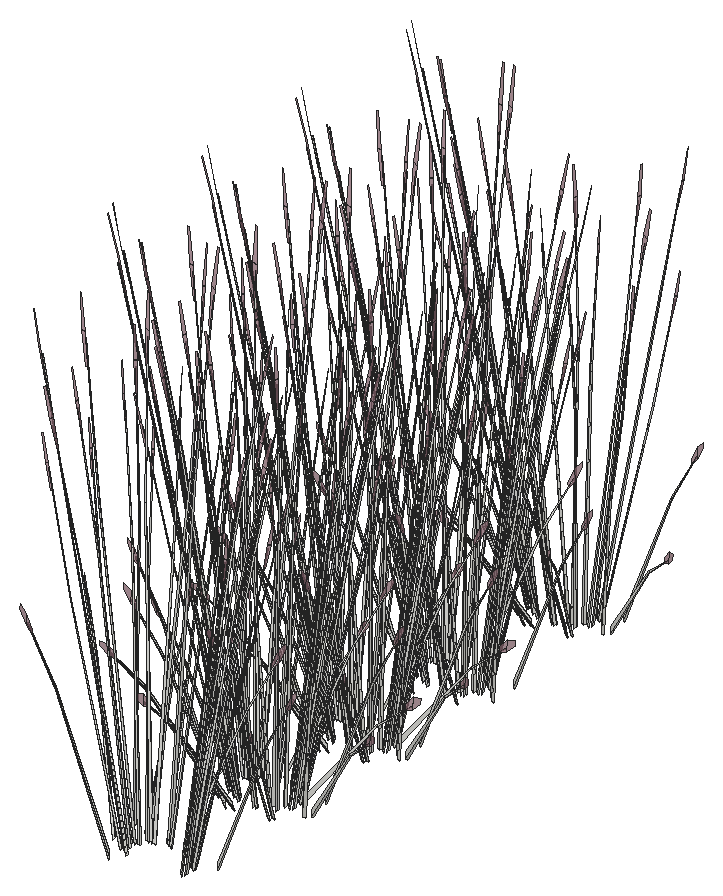
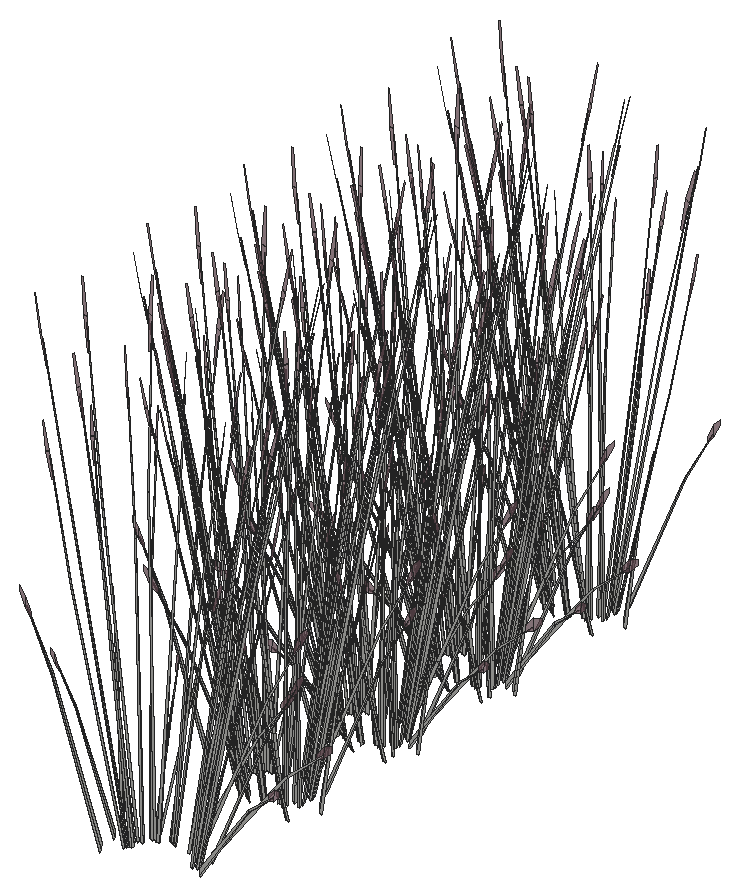
# SketchUp Ruby script. Lengths in inches.
U = 1.inch
M = Sketchup.active_model
def pt(a) = Geom::Point3d.new(a.map { |v| v * U })
def face(e, loops, mat)
  f = e.add_face(loops[0].map { |a| pt(a) })
  loops[1..].each { |l| e.add_face(l.map { |a| pt(a) }).erase! }
  f.material = f.back_material = mat if mat
  f
end
# faces: each face lists its corners as indices into pts; further lists are holes
def faces(e, pts, list, mat = nil) = list.each { |f| face(e, (f[0].is_a?(Array) ? f : [f]).map { |l| l.map { |i| pts[i] } }, mat) }
# xy, xz, yz: faces in a plane at the given z, y or x. An outline is a flat list of corners, or four numbers for a rectangle; further outlines are holes
def ring(l) = l.size == 4 ? [[l[0], l[1]], [l[2], l[1]], [l[2], l[3]], [l[0], l[3]]] : l.each_slice(2).to_a
def flat(e, list, mat, &to3) = list.each { |f| face(e, (f[0].is_a?(Array) ? f : [f]).map { |l| ring(l).map { |u, v| to3.(u, v) } }, mat) }
def xy(e, z, list, mat = nil) = flat(e, list, mat) { |x, y| [x, y, z] }
def xz(e, y, list, mat = nil) = flat(e, list, mat) { |x, z| [x, y, z] }
def yz(e, x, list, mat = nil) = flat(e, list, mat) { |y, z| [x, y, z] }
def lines(e, pts, list) = list.each { |a, b| e.add_line(pt(pts[a]), pt(pts[b])) }
# prism: a flat outline (further loops are holes) pulled along v
def prism(e, loops, v, mat = nil)
  f = face(e, loops, mat); d = Geom::Vector3d.new(v.map { |x| x * U })
  f.pushpull(f.normal.samedirection?(d) ? d.length : -d.length)
end
def box(e, o, s, mat = nil) = prism(e, [[o, [o[0] + s[0], o[1], o[2]], [o[0] + s[0], o[1] + s[1], o[2]], [o[0], o[1] + s[1], o[2]]]], [0, 0, s[2]], mat)
def at(x, y, z, deg = 0) = Geom::Transformation.translation(pt([x, y, z])) * Geom::Transformation.rotation(ORIGIN, Z_AXIS, deg.degrees)
def axes(o, x, y, z) = Geom::Transformation.new([*x, 0, *y, 0, *z, 0, *pt(o).to_a, 1])
def part(name) = M.definitions.add(name)
# library, detail: a bought-in or finely detailed component or shape, given as its bounding box
def library(name, o, s) = part(name).tap { |d| box(d.entities, o, s) }
def detail(e, o, s) = box(e.add_group.entities, o, s)
def put(e, d, t, mat = nil) = e.add_instance(d, t).tap { |i| i.material = mat if mat }
def group(e, t, mat = nil) = e.add_group.tap { |g| g.transformation = t; g.material = mat if mat }.entities
root = M.entities
M.materials.add("LightPink_Translucent").color = [144, 107, 117]
M.materials["LightPink_Translucent"].alpha = 0.75
c1 = part("blade")
p = [[2.15,0.21,22],[0,0.17,0],[0.09,0.45,0],[2.18,0.31,22],[2.29,0.31,22],[0.38,0.45,0],
  [2.48,0.24,33],[2.49,0.24,33],[2.48,0.22,33]]
faces(c1.entities,p,[[0,1,2,3],[4,5,2,3],[6,3,4,7],[8,0,3,6]])
c2 = part("seeds")
p = [[0.3,-0.1,1.38],[-0.01,-0.03,1.59],[-0.01,-0.03,0.03],[0.14,-0.07,-0.07],[0.29,-0.03,3],[0.15,0.01,3.11]]
faces(c2.entities,p,[[0,1,2,3],[1,0,4,5]],"LightPink_Translucent")
c3 = part("blade with seeds")
put(c3.entities,c1,at(0,0,0))
put(c3.entities,c2,axes([2.4,0.25,30.99],[1.5799,-0.05474,1.17369],[-0.12525,1.92788,0.29478],[-0.07173,-0.02425,1.56792]))
put(root,c3,axes([336.16,386.52,52.18],[0.34663,0.16434,0.05682],[-0.20181,0.23402,0.44729],[0.11113,-0.07566,0.68204]))
put(root,c3,axes([336.0625,386.45,52.18],[0.12522,0.35963,0.42415],[-0.49122,0.06241,0.34973],[0.14477,-0.08458,0.87768]))
put(root,c3,axes([331.47,385.46,52.16],[0.03743,0.039,1.56736],[-0.18045,0.35054,-0.1481],[-0.18276,0.00254,0.27737]))
put(root,c3,axes([332.25,386.07,52.46],[0.28729,0.24465,0.31292],[-0.32804,0.23159,-0.40398],[-0.16667,-0.03524,0.77298]))
put(root,c3,axes([335.83,387.33,52.46],[-0.41962,-0.10901,0.31292],[0.12239,-0.31802,-0.40398],[0.16894,-0.02916,0.77298]))
put(root,c3,axes([331.4375,386.75,52.18],[0.14265,-0.35629,0.42415],[0.46898,0.12183,0.34973],[-0.18443,0.02141,0.87768]))
put(root,c3,axes([331.4,386.66,52.18],[-0.18545,-0.26643,0.05682],[0.33817,-0.13041,0.44729],[-0.14907,0.02573,0.68204]))
put(root,c3,axes([336.21,387.43,52.18],[0.18545,0.26643,0.05682],[-0.33817,0.13041,0.44729],[0.14907,-0.02573,0.68204]))
put(root,c3,axes([336.18,387.34,52.18],[-0.14265,0.35629,0.42415],[-0.46898,-0.12183,0.34973],[0.18443,-0.02141,0.87768]))
put(root,c3,axes([331.78,386.76,52.46],[0.41962,0.10901,0.31292],[-0.12239,0.31802,-0.40398],[-0.16894,0.02916,0.77298]))
put(root,c3,axes([337.02,388.49,52.16],[-0.04566,-0.03421,1.56736],[0.09987,-0.36669,-0.1481],[0.17984,-0.02343,0.27737]))
put(root,c3,axes([335.36,388.02,52.46],[-0.28729,-0.24465,0.31292],[0.32804,-0.23159,-0.40398],[0.16667,0.03524,0.77298]))
put(root,c3,axes([331.55,387.64,52.18],[-0.12522,-0.35963,0.42415],[0.49122,-0.06241,0.34973],[-0.14477,0.08458,0.87768]))
put(root,c3,axes([331.45,387.57,52.18],[-0.34663,-0.16434,0.05682],[0.20181,-0.23402,0.44729],[-0.11113,0.07566,0.68204]))
put(root,c3,axes([331.85,387.52,52.46],[0.43951,-0.05584,0.31292],[0.11606,0.31924,-0.40398],[-0.12595,0.08575,0.77298]))
put(root,c3,axes([330.16,387.38,52.16],[0.06444,0.01048,1.56736],[0.19934,0.34525,-0.1481],[-0.13191,0.09062,0.27737]))
put(root,c3,axes([335.62,388.24,52.18],[-0.02542,0.29714,0.05682],[-0.38391,-0.00815,0.44729],[0.14706,0.03109,0.68204]))
put(root,c3,axes([335.65,388.15,52.18],[-0.3723,0.25748,0.42415],[-0.32109,-0.27343,0.34973],[0.17467,0.04749,0.87768]))
put(root,c3,axes([330.85,388.43,52.99],[0.44556,0.1043,-0.05733],[-0.13706,0.32103,-0.25992],[-0.07288,0.04874,0.85731]))
put(root,c3,axes([334.47,388.45,52.46],[-0.07798,-0.31474,0.31292],[0.44579,-0.08311,-0.40398],[0.11974,0.09019,0.77298]))
put(root,c3,axes([332.45,388.16,52.46],[0.34164,-0.20573,0.31292],[0.3234,0.23491,-0.40398],[-0.04921,0.11936,0.77298]))
put(root,c3,axes([334.04,388.89,52.16],[0.00149,-0.04731,1.56736],[0.4327,-0.20872,-0.1481],[0.1503,0.0745,0.27737]))
put(root,c3,axes([332.14,388.34,52.18],[-0.41493,-0.01821,0.05682],[0.01138,-0.27493,0.44729],[-0.04342,0.10531,0.68204]))
put(root,c3,axes([332.27,388.37,52.18],[-0.35954,-0.26661,0.42415],[0.38183,-0.22994,0.34973],[-0.06632,0.12508,0.87768]))
put(root,c3,axes([333.4,388.5,52.46],[0.15222,-0.30049,0.31292],[0.44409,0.08764,-0.40398],[0.04072,0.12098,0.77298]))
put(root,c3,axes([334.54,388.73,52.18],[-0.22948,0.24822,0.05682],[-0.32679,-0.14452,0.44729],[0.10565,0.07958,0.68204]))
put(root,c3,axes([334,389.57,52.99],[0.34892,-0.22417,-0.05733],[0.3197,0.24551,-0.25992],[0.02251,0.06957,0.85731]))
put(root,c3,axes([334.64,388.66,52.18],[-0.5022,0.08967,0.42415],[-0.08716,-0.35177,0.34973],[0.11811,0.10367,0.87768]))
put(root,c3,axes([333.27,388.77,52.18],[-0.37205,0.1328,0.05682],[-0.18211,-0.24217,0.44729],[0.03593,0.10675,0.68204]))
put(root,c3,axes([332.23,388.21,52.77],[0.55492,0.01936,-0.11927],[-0.01517,0.36657,-0.66198],[-0.03855,0.14118,1.00587]))
put(root,c3,axes([333.4,388.74,52.47],[-0.49753,-0.10215,0.47081],[0.17013,-0.33585,0.3882],[0.0299,0.13207,0.97422]))
put(root,c3,axes([331.05,389.18,52.16],[0.05728,-0.02359,1.56736],[0.47345,0.15692,-0.1481],[-0.01113,0.13066,0.27737]))
put(root,c3,axes([333.57,394.3,52.17],[-0.07723,-0.05479,1.54581],[-0.51538,0.03473,-0.24447],[-0.08225,-0.13104,0.12397]))
put(root,c3,axes([335.89,394.98,52.17],[-0.00487,-0.07777,1.54581],[-0.41166,-0.22476,-0.24447],[0.06364,-0.13625,0.12397]))
put(root,c3,axes([335.78,394.7,52.16],[-0.05128,0.02985,1.56736],[-0.5024,-0.1007,-0.1481],[-0.01819,-0.13025,0.27737]))
put(root,c3,axes([333.05,394.125,52.16],[-0.00942,0.04684,1.56736],[-0.46458,0.16998,-0.1481],[-0.13671,-0.08689,0.27737]))
put(root,c3,axes([332.94,394.96,52.5],[0.56246,-0.10044,0.47505],[0.09762,0.39398,0.3917],[-0.13228,-0.11611,0.983]))
put(root,c3,axes([334.22,395.03,52.18],[0.49753,0.10215,0.42415],[-0.17013,0.33585,0.34973],[-0.0299,-0.13207,0.87768]))
put(root,c3,axes([334.35,395,52.18],[0.37205,-0.1328,0.05682],[0.18211,0.24217,0.44729],[-0.03593,-0.10675,0.68204]))
put(root,c3,axes([333.07,395.04,52.18],[0.22948,-0.24822,0.05682],[0.32679,0.14452,0.44729],[-0.10565,-0.07958,0.68204]))
put(root,c3,axes([334.21,395.28,52.46],[-0.15222,0.30049,0.31292],[-0.44409,-0.08764,-0.40398],[-0.04072,-0.12098,0.77298]))
put(root,c3,axes([335.34,395.4,52.18],[0.35954,0.26661,0.42415],[-0.38183,0.22994,0.34973],[0.06632,-0.12508,0.87768]))
put(root,c3,axes([333.18,395.02,52.8],[-0.33698,0.3746,-0.12034],[-0.48801,-0.21581,-0.66795],[-0.16964,-0.10584,1.01494]))
put(root,c3,axes([335.48,395.43,52.18],[0.41493,0.01821,0.05682],[-0.01138,0.27493,0.44729],[0.04342,-0.10531,0.68204]))
put(root,c3,axes([335.17,395.62,52.46],[-0.34164,0.20573,0.31292],[-0.3234,-0.23491,-0.40398],[0.04921,-0.11936,0.77298]))
put(root,c3,axes([331.88,394.91,52.17],[-0.10864,-0.00276,1.54581],[-0.34587,0.27582,-0.24447],[-0.18454,-0.05636,0.12397]))
put(root,c3,axes([333.14,395.33,52.46],[0.07798,0.31474,0.31292],[-0.44579,0.08311,-0.40398],[-0.11974,-0.09019,0.77298]))
put(root,c3,axes([331.8,395.53,52.5],[0.41698,-0.28837,0.47505],[0.35962,0.30624,0.3917],[-0.19563,-0.05319,0.983]))
put(root,c3,axes([337.14,396.1875,52.16],[-0.06595,-0.00297,1.56736],[-0.27386,-0.31799,-0.1481],[0.10998,-0.10455,0.27737]))
put(root,c3,axes([331.99,395.53,52.18],[0.02542,-0.29714,0.05682],[0.38391,0.00815,0.44729],[-0.14706,-0.03109,0.68204]))
put(root,c3,axes([335.76,396.25,52.46],[-0.43951,0.05584,0.31292],[-0.11606,-0.31924,-0.40398],[0.12595,-0.08575,0.77298]))
put(root,c3,axes([336.16,396.2,52.18],[0.34663,0.16434,0.05682],[-0.20181,0.23402,0.44729],[0.11113,-0.07566,0.68204]))
put(root,c3,axes([336.0625,396.13,52.18],[0.12522,0.35963,0.42415],[-0.49122,0.06241,0.34973],[0.14477,-0.08458,0.87768]))
put(root,c3,axes([337.39,396.57,52.17],[0.07006,-0.05952,1.54581],[-0.08968,-0.3651,-0.24447],[0.1758,-0.06922,0.12397]))
put(root,c3,axes([331.47,395.14,52.16],[0.03743,0.039,1.56736],[-0.18045,0.35054,-0.1481],[-0.18276,0.00254,0.27737]))
put(root,c3,axes([332.25,395.75,52.46],[0.28729,0.24465,0.31292],[-0.32804,0.23159,-0.40398],[-0.16667,-0.03524,0.77298]))
put(root,c3,axes([335.83,397.01,52.46],[-0.41962,-0.10901,0.31292],[0.12239,-0.31802,-0.40398],[0.16894,-0.02916,0.77298]))
put(root,c3,axes([331.4375,396.43,52.18],[0.14265,-0.35629,0.42415],[0.46898,0.12183,0.34973],[-0.18443,0.02141,0.87768]))
put(root,c3,axes([331.4,396.34,52.18],[-0.18545,-0.26643,0.05682],[0.33817,-0.13041,0.44729],[-0.14907,0.02573,0.68204]))
put(root,c3,axes([336.21,397.11,52.18],[0.18545,0.26643,0.05682],[-0.33817,0.13041,0.44729],[0.14907,-0.02573,0.68204]))
put(root,c3,axes([336.18,397.02,52.18],[-0.14265,0.35629,0.42415],[-0.46898,-0.12183,0.34973],[0.18443,-0.02141,0.87768]))
put(root,c3,axes([331.78,396.4375,52.46],[0.41962,0.10901,0.31292],[-0.12239,0.31802,-0.40398],[-0.16894,0.02916,0.77298]))
put(root,c3,axes([337.02,398.17,52.16],[-0.04566,-0.03421,1.56736],[0.09987,-0.36669,-0.1481],[0.17984,-0.02343,0.27737]))
put(root,c3,axes([331.08,396.68,52.17],[-0.08245,0.05073,1.54581],[0.00701,0.37067,-0.24447],[-0.18899,0.0482,0.12397]))
put(root,c3,axes([335.36,397.7,52.46],[-0.28729,-0.24465,0.31292],[0.32804,-0.23159,-0.40398],[0.16667,0.03524,0.77298]))
put(root,c3,axes([335.88,397.62,52.17],[0.10831,-0.00661,1.54581],[0.29709,-0.30358,-0.24447],[0.19266,0.04007,0.12397]))
put(root,c3,axes([331.55,397.32,52.18],[-0.12522,-0.35963,0.42415],[0.49122,-0.06241,0.34973],[-0.14477,0.08458,0.87768]))
put(root,c3,axes([331.45,397.25,52.18],[-0.34663,-0.16434,0.05682],[0.20181,-0.23402,0.44729],[-0.11113,0.07566,0.68204]))
put(root,c3,axes([331.85,397.2,52.46],[0.43951,-0.05584,0.31292],[0.11606,0.31924,-0.40398],[-0.12595,0.08575,0.77298]))
put(root,c3,axes([330.16,397.06,52.16],[0.06444,0.01048,1.56736],[0.19934,0.34525,-0.1481],[-0.13191,0.09062,0.27737]))
put(root,c3,axes([335.62,397.92,52.18],[-0.02542,0.29714,0.05682],[-0.38391,-0.00815,0.44729],[0.14706,0.03109,0.68204]))
put(root,c3,axes([335.65,397.83,52.18],[-0.3723,0.25748,0.42415],[-0.32109,-0.27343,0.34973],[0.17467,0.04749,0.87768]))
put(root,c3,axes([330.85,398.11,52.99],[0.44556,0.1043,-0.05733],[-0.13706,0.32103,-0.25992],[-0.07288,0.04874,0.85731]))
put(root,c3,axes([334.47,398.125,52.46],[-0.07798,-0.31474,0.31292],[0.44579,-0.08311,-0.40398],[0.11974,0.09019,0.77298]))
put(root,c3,axes([332.45,397.84,52.46],[0.34164,-0.20573,0.31292],[0.3234,0.23491,-0.40398],[-0.04921,0.11936,0.77298]))
put(root,c3,axes([334.04,398.57,52.16],[0.00149,-0.04731,1.56736],[0.4327,-0.20872,-0.1481],[0.1503,0.0745,0.27737]))
put(root,c3,axes([332.14,398.02,52.18],[-0.41493,-0.01821,0.05682],[0.01138,-0.27493,0.44729],[-0.04342,0.10531,0.68204]))
put(root,c3,axes([332.27,398.05,52.18],[-0.35954,-0.26661,0.42415],[0.38183,-0.22994,0.34973],[-0.06632,0.12508,0.87768]))
put(root,c3,axes([333.4,398.18,52.46],[0.15222,-0.30049,0.31292],[0.44409,0.08764,-0.40398],[0.04072,0.12098,0.77298]))
put(root,c3,axes([334.54,398.41,52.18],[-0.22948,0.24822,0.05682],[-0.32679,-0.14452,0.44729],[0.10565,0.07958,0.68204]))
put(root,c3,axes([334,399.25,52.99],[0.34892,-0.22417,-0.05733],[0.3197,0.24551,-0.25992],[0.02251,0.06957,0.85731]))
put(root,c3,axes([334.64,398.34,52.18],[-0.5022,0.08967,0.42415],[-0.08716,-0.35177,0.34973],[0.11811,0.10367,0.87768]))
put(root,c3,axes([333.57,402.77,52.17],[-0.07723,-0.05479,1.54581],[-0.51538,0.03473,-0.24447],[-0.08225,-0.13104,0.12397]))
put(root,c3,axes([333.27,398.45,52.18],[-0.37205,0.1328,0.05682],[-0.18211,-0.24217,0.44729],[0.03593,0.10675,0.68204]))
put(root,c3,axes([331.09,398.07,52.17],[-0.01255,0.07733,1.54581],[0.35618,0.269,-0.24447],[-0.09325,0.12721,0.12397]))
put(root,c3,axes([332.23,397.89,52.77],[0.55492,0.01936,-0.11927],[-0.01517,0.36657,-0.66198],[-0.03855,0.14118,1.00587]))
put(root,c3,axes([333.4,398.42,52.47],[-0.49753,-0.10215,0.47081],[0.17013,-0.33585,0.3882],[0.0299,0.13207,0.97422]))
put(root,c3,axes([335.89,403.4375,52.17],[-0.00487,-0.07777,1.54581],[-0.41166,-0.22476,-0.24447],[0.06364,-0.13625,0.12397]))
put(root,c3,axes([335.78,403.16,52.16],[-0.05128,0.02985,1.56736],[-0.5024,-0.1007,-0.1481],[-0.01819,-0.13025,0.27737]))
put(root,c3,axes([333.05,402.59,52.16],[-0.00942,0.04684,1.56736],[-0.46458,0.16998,-0.1481],[-0.13671,-0.08689,0.27737]))
put(root,c3,axes([331.05,398.86,52.16],[0.05728,-0.02359,1.56736],[0.47345,0.15692,-0.1481],[-0.01113,0.13066,0.27737]))
put(root,c3,axes([332.94,403.42,52.5],[0.56246,-0.10044,0.47505],[0.09762,0.39398,0.3917],[-0.13228,-0.11611,0.983]))
put(root,c3,axes([334.22,403.49,52.18],[0.49753,0.10215,0.42415],[-0.17013,0.33585,0.34973],[-0.0299,-0.13207,0.87768]))
put(root,c3,axes([334.35,403.47,52.18],[0.37205,-0.1328,0.05682],[0.18211,0.24217,0.44729],[-0.03593,-0.10675,0.68204]))
put(root,c3,axes([333.14,399.03,52.17],[0.064,0.06292,1.54581],[0.51651,0.02472,-0.24447],[0.05194,0.13877,0.12397]))
put(root,c3,axes([333.07,403.5,52.18],[0.22948,-0.24822,0.05682],[0.32679,0.14452,0.44729],[-0.10565,-0.07958,0.68204]))
put(root,c3,axes([334.21,403.74,52.46],[-0.15222,0.30049,0.31292],[-0.44409,-0.08764,-0.40398],[-0.04072,-0.12098,0.77298]))
put(root,c3,axes([335.34,403.87,52.18],[0.35954,0.26661,0.42415],[-0.38183,0.22994,0.34973],[0.06632,-0.12508,0.87768]))
put(root,c3,axes([333.18,403.48,52.8],[-0.33698,0.3746,-0.12034],[-0.48801,-0.21581,-0.66795],[-0.16964,-0.10584,1.01494]))
put(root,c3,axes([335.48,403.89,52.18],[0.41493,0.01821,0.05682],[-0.01138,0.27493,0.44729],[0.04342,-0.10531,0.68204]))
put(root,c3,axes([335.17,404.08,52.46],[-0.34164,0.20573,0.31292],[-0.3234,-0.23491,-0.40398],[0.04921,-0.11936,0.77298]))
put(root,c3,axes([331.88,403.37,52.17],[-0.10864,-0.00276,1.54581],[-0.34587,0.27582,-0.24447],[-0.18454,-0.05636,0.12397]))
put(root,c3,axes([333.14,403.79,52.46],[0.07798,0.31474,0.31292],[-0.44579,0.08311,-0.40398],[-0.11974,-0.09019,0.77298]))
put(root,c3,axes([331.8,403.99,52.5],[0.41698,-0.28837,0.47505],[0.35962,0.30624,0.3917],[-0.19563,-0.05319,0.983]))
put(root,c3,axes([337.14,404.65,52.16],[-0.06595,-0.00297,1.56736],[-0.27386,-0.31799,-0.1481],[0.10998,-0.10455,0.27737]))
put(root,c3,axes([331.99,403.99,52.18],[0.02542,-0.29714,0.05682],[0.38391,0.00815,0.44729],[-0.14706,-0.03109,0.68204]))
put(root,c3,axes([335.76,404.71,52.46],[-0.43951,0.05584,0.31292],[-0.11606,-0.31924,-0.40398],[0.12595,-0.08575,0.77298]))
put(root,c3,axes([336.16,404.66,52.18],[0.34663,0.16434,0.05682],[-0.20181,0.23402,0.44729],[0.11113,-0.07566,0.68204]))
put(root,c3,axes([336.0625,404.59,52.18],[0.12522,0.35963,0.42415],[-0.49122,0.06241,0.34973],[0.14477,-0.08458,0.87768]))
put(root,c3,axes([337.39,405.03,52.17],[0.07006,-0.05952,1.54581],[-0.08968,-0.3651,-0.24447],[0.1758,-0.06922,0.12397]))
put(root,c3,axes([331.47,403.6,52.16],[0.03743,0.039,1.56736],[-0.18045,0.35054,-0.1481],[-0.18276,0.00254,0.27737]))
put(root,c3,axes([332.25,404.21,52.46],[0.28729,0.24465,0.31292],[-0.32804,0.23159,-0.40398],[-0.16667,-0.03524,0.77298]))
put(root,c3,axes([335.83,405.48,52.46],[-0.41962,-0.10901,0.31292],[0.12239,-0.31802,-0.40398],[0.16894,-0.02916,0.77298]))
put(root,c3,axes([331.4375,404.9,52.18],[0.14265,-0.35629,0.42415],[0.46898,0.12183,0.34973],[-0.18443,0.02141,0.87768]))
put(root,c3,axes([331.4,404.8,52.18],[-0.18545,-0.26643,0.05682],[0.33817,-0.13041,0.44729],[-0.14907,0.02573,0.68204]))
put(root,c3,axes([336.21,405.58,52.18],[0.18545,0.26643,0.05682],[-0.33817,0.13041,0.44729],[0.14907,-0.02573,0.68204]))
put(root,c3,axes([336.18,405.48,52.18],[-0.14265,0.35629,0.42415],[-0.46898,-0.12183,0.34973],[0.18443,-0.02141,0.87768]))
put(root,c3,axes([331.78,404.9,52.46],[0.41962,0.10901,0.31292],[-0.12239,0.31802,-0.40398],[-0.16894,0.02916,0.77298]))
put(root,c3,axes([337.02,406.63,52.16],[-0.04566,-0.03421,1.56736],[0.09987,-0.36669,-0.1481],[0.17984,-0.02343,0.27737]))
put(root,c3,axes([331.08,405.15,52.17],[-0.08245,0.05073,1.54581],[0.00701,0.37067,-0.24447],[-0.18899,0.0482,0.12397]))
put(root,c3,axes([335.36,406.16,52.46],[-0.28729,-0.24465,0.31292],[0.32804,-0.23159,-0.40398],[0.16667,0.03524,0.77298]))
put(root,c3,axes([335.88,406.08,52.17],[0.10831,-0.00661,1.54581],[0.29709,-0.30358,-0.24447],[0.19266,0.04007,0.12397]))
put(root,c3,axes([331.55,405.78,52.18],[-0.12522,-0.35963,0.42415],[0.49122,-0.06241,0.34973],[-0.14477,0.08458,0.87768]))
put(root,c3,axes([331.45,405.71,52.18],[-0.34663,-0.16434,0.05682],[0.20181,-0.23402,0.44729],[-0.11113,0.07566,0.68204]))
put(root,c3,axes([331.85,405.66,52.46],[0.43951,-0.05584,0.31292],[0.11606,0.31924,-0.40398],[-0.12595,0.08575,0.77298]))
put(root,c3,axes([330.16,405.52,52.16],[0.06444,0.01048,1.56736],[0.19934,0.34525,-0.1481],[-0.13191,0.09062,0.27737]))
put(root,c3,axes([335.62,406.38,52.18],[-0.02542,0.29714,0.05682],[-0.38391,-0.00815,0.44729],[0.14706,0.03109,0.68204]))
put(root,c3,axes([335.65,406.29,52.18],[-0.3723,0.25748,0.42415],[-0.32109,-0.27343,0.34973],[0.17467,0.04749,0.87768]))
put(root,c3,axes([330.85,406.57,52.99],[0.44556,0.1043,-0.05733],[-0.13706,0.32103,-0.25992],[-0.07288,0.04874,0.85731]))
put(root,c3,axes([334.47,406.59,52.46],[-0.07798,-0.31474,0.31292],[0.44579,-0.08311,-0.40398],[0.11974,0.09019,0.77298]))
put(root,c3,axes([332.45,406.3,52.46],[0.34164,-0.20573,0.31292],[0.3234,0.23491,-0.40398],[-0.04921,0.11936,0.77298]))
put(root,c3,axes([334.04,407.03,52.16],[0.00149,-0.04731,1.56736],[0.4327,-0.20872,-0.1481],[0.1503,0.0745,0.27737]))
put(root,c3,axes([332.14,406.49,52.18],[-0.41493,-0.01821,0.05682],[0.01138,-0.27493,0.44729],[-0.04342,0.10531,0.68204]))
put(root,c3,axes([332.27,406.51,52.18],[-0.35954,-0.26661,0.42415],[0.38183,-0.22994,0.34973],[-0.06632,0.12508,0.87768]))
put(root,c3,axes([333.4,406.64,52.46],[0.15222,-0.30049,0.31292],[0.44409,0.08764,-0.40398],[0.04072,0.12098,0.77298]))
put(root,c3,axes([334.54,406.87,52.18],[-0.22948,0.24822,0.05682],[-0.32679,-0.14452,0.44729],[0.10565,0.07958,0.68204]))
put(root,c3,axes([334,407.71,52.99],[0.34892,-0.22417,-0.05733],[0.3197,0.24551,-0.25992],[0.02251,0.06957,0.85731]))
put(root,c3,axes([334.64,406.8,52.18],[-0.5022,0.08967,0.42415],[-0.08716,-0.35177,0.34973],[0.11811,0.10367,0.87768]))
put(root,c3,axes([333.27,406.91,52.18],[-0.37205,0.1328,0.05682],[-0.18211,-0.24217,0.44729],[0.03593,0.10675,0.68204]))
put(root,c3,axes([331.09,406.53,52.17],[-0.01255,0.07733,1.54581],[0.35618,0.269,-0.24447],[-0.09325,0.12721,0.12397]))
put(root,c3,axes([332.23,406.36,52.77],[0.55492,0.01936,-0.11927],[-0.01517,0.36657,-0.66198],[-0.03855,0.14118,1.00587]))
put(root,c3,axes([333.4,406.88,52.47],[-0.49753,-0.10215,0.47081],[0.17013,-0.33585,0.3882],[0.0299,0.13207,0.97422]))
put(root,c3,axes([335.78,411.625,52.16],[-0.05128,0.02985,1.56736],[-0.5024,-0.1007,-0.1481],[-0.01819,-0.13025,0.27737]))
put(root,c3,axes([333.05,411.05,52.16],[-0.00942,0.04684,1.56736],[-0.46458,0.16998,-0.1481],[-0.13671,-0.08689,0.27737]))
put(root,c3,axes([331.05,407.32,52.16],[0.05728,-0.02359,1.56736],[0.47345,0.15692,-0.1481],[-0.01113,0.13066,0.27737]))
put(root,c3,axes([332.94,411.88,52.5],[0.56246,-0.10044,0.47505],[0.09762,0.39398,0.3917],[-0.13228,-0.11611,0.983]))
put(root,c3,axes([334.22,411.96,52.18],[0.49753,0.10215,0.42415],[-0.17013,0.33585,0.34973],[-0.0299,-0.13207,0.87768]))
put(root,c3,axes([334.35,411.93,52.18],[0.37205,-0.1328,0.05682],[0.18211,0.24217,0.44729],[-0.03593,-0.10675,0.68204]))
put(root,c3,axes([333.14,407.49,52.17],[0.064,0.06292,1.54581],[0.51651,0.02472,-0.24447],[0.05194,0.13877,0.12397]))
put(root,c3,axes([333.07,411.97,52.18],[0.22948,-0.24822,0.05682],[0.32679,0.14452,0.44729],[-0.10565,-0.07958,0.68204]))
put(root,c3,axes([334.21,412.2,52.46],[-0.15222,0.30049,0.31292],[-0.44409,-0.08764,-0.40398],[-0.04072,-0.12098,0.77298]))
put(root,c3,axes([335.34,412.33,52.18],[0.35954,0.26661,0.42415],[-0.38183,0.22994,0.34973],[0.06632,-0.12508,0.87768]))
put(root,c3,axes([333.18,411.94,52.8],[-0.33698,0.3746,-0.12034],[-0.48801,-0.21581,-0.66795],[-0.16964,-0.10584,1.01494]))
put(root,c3,axes([335.48,412.36,52.18],[0.41493,0.01821,0.05682],[-0.01138,0.27493,0.44729],[0.04342,-0.10531,0.68204]))
put(root,c3,axes([335.17,412.54,52.46],[-0.34164,0.20573,0.31292],[-0.3234,-0.23491,-0.40398],[0.04921,-0.11936,0.77298]))
put(root,c3,axes([333.14,412.25,52.46],[0.07798,0.31474,0.31292],[-0.44579,0.08311,-0.40398],[-0.11974,-0.09019,0.77298]))
put(root,c3,axes([331.8,412.46,52.5],[0.41698,-0.28837,0.47505],[0.35962,0.30624,0.3917],[-0.19563,-0.05319,0.983]))
put(root,c3,axes([337.14,413.11,52.16],[-0.06595,-0.00297,1.56736],[-0.27386,-0.31799,-0.1481],[0.10998,-0.10455,0.27737]))
put(root,c3,axes([331.99,412.46,52.18],[0.02542,-0.29714,0.05682],[0.38391,0.00815,0.44729],[-0.14706,-0.03109,0.68204]))
put(root,c3,axes([335.76,413.18,52.46],[-0.43951,0.05584,0.31292],[-0.11606,-0.31924,-0.40398],[0.12595,-0.08575,0.77298]))
put(root,c3,axes([336.16,413.13,52.18],[0.34663,0.16434,0.05682],[-0.20181,0.23402,0.44729],[0.11113,-0.07566,0.68204]))
put(root,c3,axes([336.0625,413.06,52.18],[0.12522,0.35963,0.42415],[-0.49122,0.06241,0.34973],[0.14477,-0.08458,0.87768]))
put(root,c3,axes([331.47,412.07,52.16],[0.03743,0.039,1.56736],[-0.18045,0.35054,-0.1481],[-0.18276,0.00254,0.27737]))
put(root,c3,axes([332.25,412.68,52.46],[0.28729,0.24465,0.31292],[-0.32804,0.23159,-0.40398],[-0.16667,-0.03524,0.77298]))
put(root,c3,axes([335.83,413.94,52.46],[-0.41962,-0.10901,0.31292],[0.12239,-0.31802,-0.40398],[0.16894,-0.02916,0.77298]))
put(root,c3,axes([331.4375,413.36,52.18],[0.14265,-0.35629,0.42415],[0.46898,0.12183,0.34973],[-0.18443,0.02141,0.87768]))
put(root,c3,axes([331.4,413.27,52.18],[-0.18545,-0.26643,0.05682],[0.33817,-0.13041,0.44729],[-0.14907,0.02573,0.68204]))
put(root,c3,axes([336.21,414.04,52.18],[0.18545,0.26643,0.05682],[-0.33817,0.13041,0.44729],[0.14907,-0.02573,0.68204]))
put(root,c3,axes([336.18,413.95,52.18],[-0.14265,0.35629,0.42415],[-0.46898,-0.12183,0.34973],[0.18443,-0.02141,0.87768]))
put(root,c3,axes([331.78,413.37,52.46],[0.41962,0.10901,0.31292],[-0.12239,0.31802,-0.40398],[-0.16894,0.02916,0.77298]))
put(root,c3,axes([337.02,415.1,52.16],[-0.04566,-0.03421,1.56736],[0.09987,-0.36669,-0.1481],[0.17984,-0.02343,0.27737]))
put(root,c3,axes([335.36,414.63,52.46],[-0.28729,-0.24465,0.31292],[0.32804,-0.23159,-0.40398],[0.16667,0.03524,0.77298]))
put(root,c3,axes([331.55,414.25,52.18],[-0.12522,-0.35963,0.42415],[0.49122,-0.06241,0.34973],[-0.14477,0.08458,0.87768]))
put(root,c3,axes([331.45,414.18,52.18],[-0.34663,-0.16434,0.05682],[0.20181,-0.23402,0.44729],[-0.11113,0.07566,0.68204]))
put(root,c3,axes([331.85,414.13,52.46],[0.43951,-0.05584,0.31292],[0.11606,0.31924,-0.40398],[-0.12595,0.08575,0.77298]))
put(root,c3,axes([330.16,413.99,52.16],[0.06444,0.01048,1.56736],[0.19934,0.34525,-0.1481],[-0.13191,0.09062,0.27737]))
put(root,c3,axes([335.62,414.85,52.18],[-0.02542,0.29714,0.05682],[-0.38391,-0.00815,0.44729],[0.14706,0.03109,0.68204]))
put(root,c3,axes([335.65,414.76,52.18],[-0.3723,0.25748,0.42415],[-0.32109,-0.27343,0.34973],[0.17467,0.04749,0.87768]))
put(root,c3,axes([330.85,415.04,52.99],[0.44556,0.1043,-0.05733],[-0.13706,0.32103,-0.25992],[-0.07288,0.04874,0.85731]))
put(root,c3,axes([334.47,415.05,52.46],[-0.07798,-0.31474,0.31292],[0.44579,-0.08311,-0.40398],[0.11974,0.09019,0.77298]))
put(root,c3,axes([332.45,414.77,52.46],[0.34164,-0.20573,0.31292],[0.3234,0.23491,-0.40398],[-0.04921,0.11936,0.77298]))
put(root,c3,axes([334.04,415.49,52.16],[0.00149,-0.04731,1.56736],[0.4327,-0.20872,-0.1481],[0.1503,0.0745,0.27737]))
put(root,c3,axes([332.14,414.95,52.18],[-0.41493,-0.01821,0.05682],[0.01138,-0.27493,0.44729],[-0.04342,0.10531,0.68204]))
put(root,c3,axes([332.27,414.98,52.18],[-0.35954,-0.26661,0.42415],[0.38183,-0.22994,0.34973],[-0.06632,0.12508,0.87768]))
put(root,c3,axes([333.4,415.1,52.46],[0.15222,-0.30049,0.31292],[0.44409,0.08764,-0.40398],[0.04072,0.12098,0.77298]))
put(root,c3,axes([334.54,415.34,52.18],[-0.22948,0.24822,0.05682],[-0.32679,-0.14452,0.44729],[0.10565,0.07958,0.68204]))
put(root,c3,axes([334,416.18,52.99],[0.34892,-0.22417,-0.05733],[0.3197,0.24551,-0.25992],[0.02251,0.06957,0.85731]))
put(root,c3,axes([334.64,415.27,52.18],[-0.5022,0.08967,0.42415],[-0.08716,-0.35177,0.34973],[0.11811,0.10367,0.87768]))
put(root,c3,axes([333.27,415.375,52.18],[-0.37205,0.1328,0.05682],[-0.18211,-0.24217,0.44729],[0.03593,0.10675,0.68204]))
put(root,c3,axes([332.23,414.82,52.77],[0.55492,0.01936,-0.11927],[-0.01517,0.36657,-0.66198],[-0.03855,0.14118,1.00587]))
put(root,c3,axes([333.4,415.35,52.47],[-0.49753,-0.10215,0.47081],[0.17013,-0.33585,0.3882],[0.0299,0.13207,0.97422]))
put(root,c3,axes([331.05,415.79,52.16],[0.05728,-0.02359,1.56736],[0.47345,0.15692,-0.1481],[-0.01113,0.13066,0.27737]))
put(root,c3,axes([333.57,421.13,52.17],[-0.07723,-0.05479,1.54581],[-0.51538,0.03473,-0.24447],[-0.08225,-0.13104,0.12397]))
put(root,c3,axes([335.89,421.8,52.17],[-0.00487,-0.07777,1.54581],[-0.41166,-0.22476,-0.24447],[0.06364,-0.13625,0.12397]))
put(root,c3,axes([335.78,421.52,52.16],[-0.05128,0.02985,1.56736],[-0.5024,-0.1007,-0.1481],[-0.01819,-0.13025,0.27737]))
put(root,c3,axes([333.05,420.95,52.16],[-0.00942,0.04684,1.56736],[-0.46458,0.16998,-0.1481],[-0.13671,-0.08689,0.27737]))
put(root,c3,axes([332.94,421.78,52.5],[0.56246,-0.10044,0.47505],[0.09762,0.39398,0.3917],[-0.13228,-0.11611,0.983]))
put(root,c3,axes([334.22,421.86,52.18],[0.49753,0.10215,0.42415],[-0.17013,0.33585,0.34973],[-0.0299,-0.13207,0.87768]))
put(root,c3,axes([334.35,421.83,52.18],[0.37205,-0.1328,0.05682],[0.18211,0.24217,0.44729],[-0.03593,-0.10675,0.68204]))
put(root,c3,axes([333.07,421.87,52.18],[0.22948,-0.24822,0.05682],[0.32679,0.14452,0.44729],[-0.10565,-0.07958,0.68204]))
put(root,c3,axes([334.21,422.1,52.46],[-0.15222,0.30049,0.31292],[-0.44409,-0.08764,-0.40398],[-0.04072,-0.12098,0.77298]))
put(root,c3,axes([335.34,422.23,52.18],[0.35954,0.26661,0.42415],[-0.38183,0.22994,0.34973],[0.06632,-0.12508,0.87768]))
put(root,c3,axes([333.18,421.84,52.8],[-0.33698,0.3746,-0.12034],[-0.48801,-0.21581,-0.66795],[-0.16964,-0.10584,1.01494]))
put(root,c3,axes([335.48,422.25,52.18],[0.41493,0.01821,0.05682],[-0.01138,0.27493,0.44729],[0.04342,-0.10531,0.68204]))
put(root,c3,axes([335.17,422.44,52.46],[-0.34164,0.20573,0.31292],[-0.3234,-0.23491,-0.40398],[0.04921,-0.11936,0.77298]))
put(root,c3,axes([331.88,421.73,52.17],[-0.10864,-0.00276,1.54581],[-0.34587,0.27582,-0.24447],[-0.18454,-0.05636,0.12397]))
put(root,c3,axes([333.14,422.15,52.46],[0.07798,0.31474,0.31292],[-0.44579,0.08311,-0.40398],[-0.11974,-0.09019,0.77298]))
put(root,c3,axes([331.8,422.36,52.5],[0.41698,-0.28837,0.47505],[0.35962,0.30624,0.3917],[-0.19563,-0.05319,0.983]))
put(root,c3,axes([337.14,423.01,52.16],[-0.06595,-0.00297,1.56736],[-0.27386,-0.31799,-0.1481],[0.10998,-0.10455,0.27737]))
put(root,c3,axes([331.99,422.36,52.18],[0.02542,-0.29714,0.05682],[0.38391,0.00815,0.44729],[-0.14706,-0.03109,0.68204]))
put(root,c3,axes([335.76,423.08,52.46],[-0.43951,0.05584,0.31292],[-0.11606,-0.31924,-0.40398],[0.12595,-0.08575,0.77298]))
put(root,c3,axes([336.16,423.03,52.18],[0.34663,0.16434,0.05682],[-0.20181,0.23402,0.44729],[0.11113,-0.07566,0.68204]))
put(root,c3,axes([336.0625,422.96,52.18],[0.12522,0.35963,0.42415],[-0.49122,0.06241,0.34973],[0.14477,-0.08458,0.87768]))
put(root,c3,axes([337.39,423.39,52.17],[0.07006,-0.05952,1.54581],[-0.08968,-0.3651,-0.24447],[0.1758,-0.06922,0.12397]))
put(root,c3,axes([331.47,421.97,52.16],[0.03743,0.039,1.56736],[-0.18045,0.35054,-0.1481],[-0.18276,0.00254,0.27737]))
put(root,c3,axes([332.25,422.58,52.46],[0.28729,0.24465,0.31292],[-0.32804,0.23159,-0.40398],[-0.16667,-0.03524,0.77298]))
put(root,c3,axes([335.83,423.84,52.46],[-0.41962,-0.10901,0.31292],[0.12239,-0.31802,-0.40398],[0.16894,-0.02916,0.77298]))
put(root,c3,axes([331.4375,423.26,52.18],[0.14265,-0.35629,0.42415],[0.46898,0.12183,0.34973],[-0.18443,0.02141,0.87768]))
put(root,c3,axes([331.4,423.16,52.18],[-0.18545,-0.26643,0.05682],[0.33817,-0.13041,0.44729],[-0.14907,0.02573,0.68204]))
put(root,c3,axes([336.21,423.9375,52.18],[0.18545,0.26643,0.05682],[-0.33817,0.13041,0.44729],[0.14907,-0.02573,0.68204]))
put(root,c3,axes([336.18,423.84,52.18],[-0.14265,0.35629,0.42415],[-0.46898,-0.12183,0.34973],[0.18443,-0.02141,0.87768]))
put(root,c3,axes([331.78,423.26,52.46],[0.41962,0.10901,0.31292],[-0.12239,0.31802,-0.40398],[-0.16894,0.02916,0.77298]))
put(root,c3,axes([337.02,425,52.16],[-0.04566,-0.03421,1.56736],[0.09987,-0.36669,-0.1481],[0.17984,-0.02343,0.27737]))
put(root,c3,axes([331.08,423.51,52.17],[-0.08245,0.05073,1.54581],[0.00701,0.37067,-0.24447],[-0.18899,0.0482,0.12397]))
